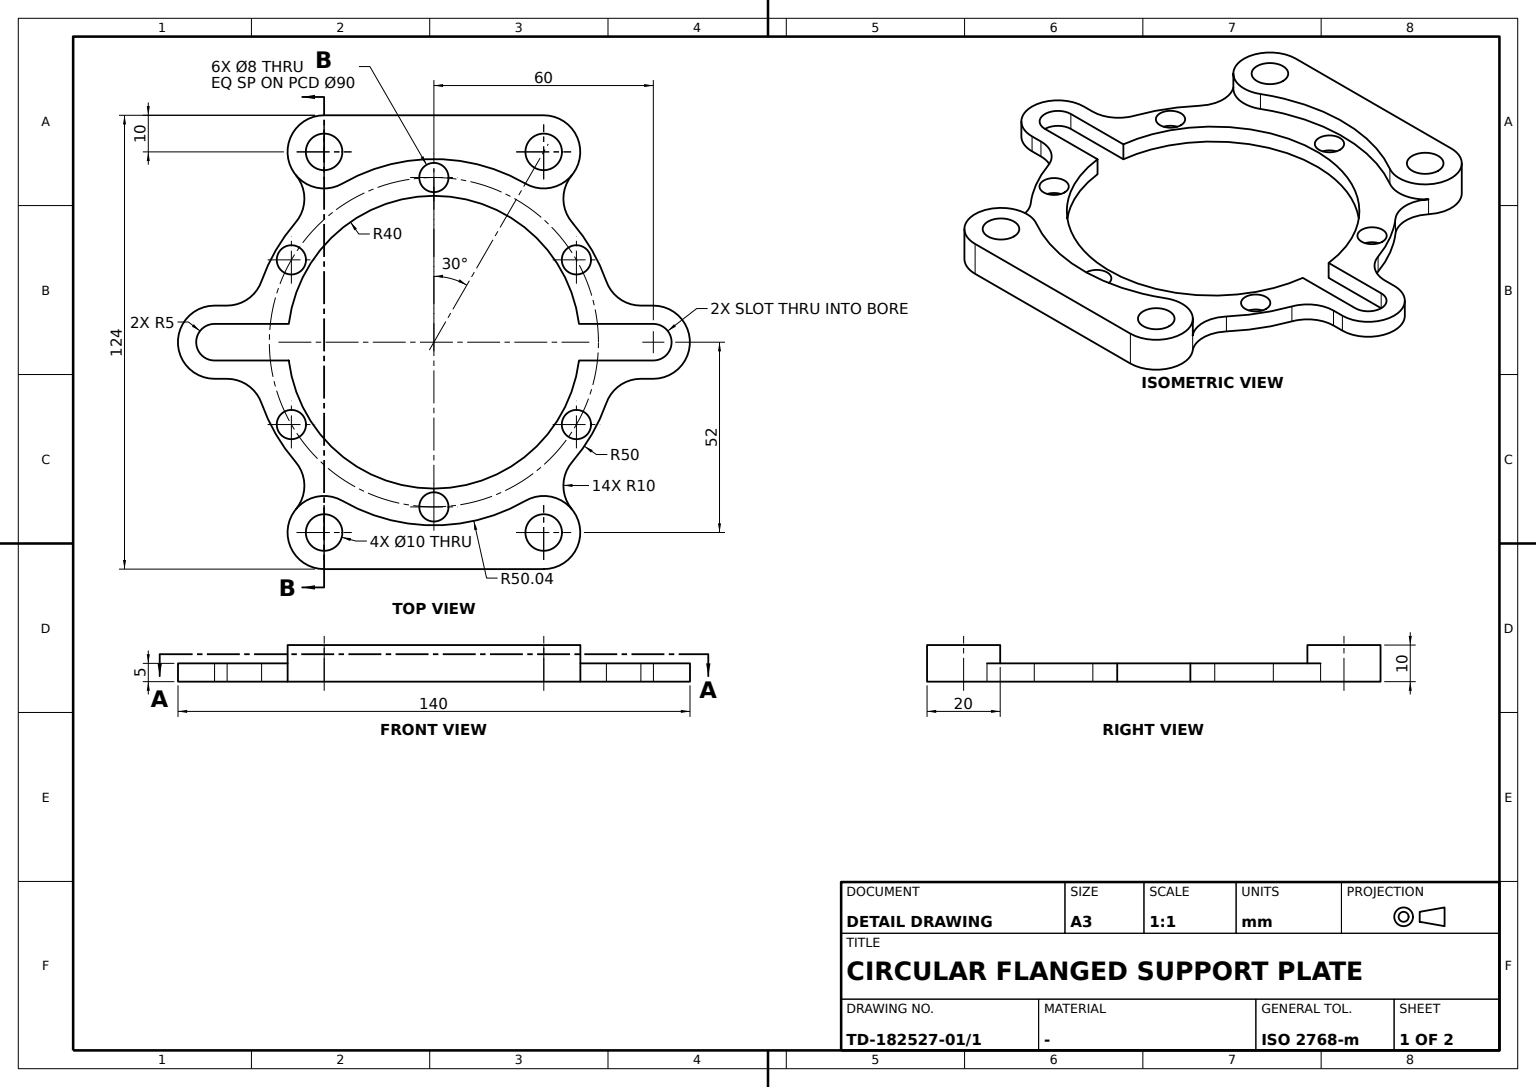
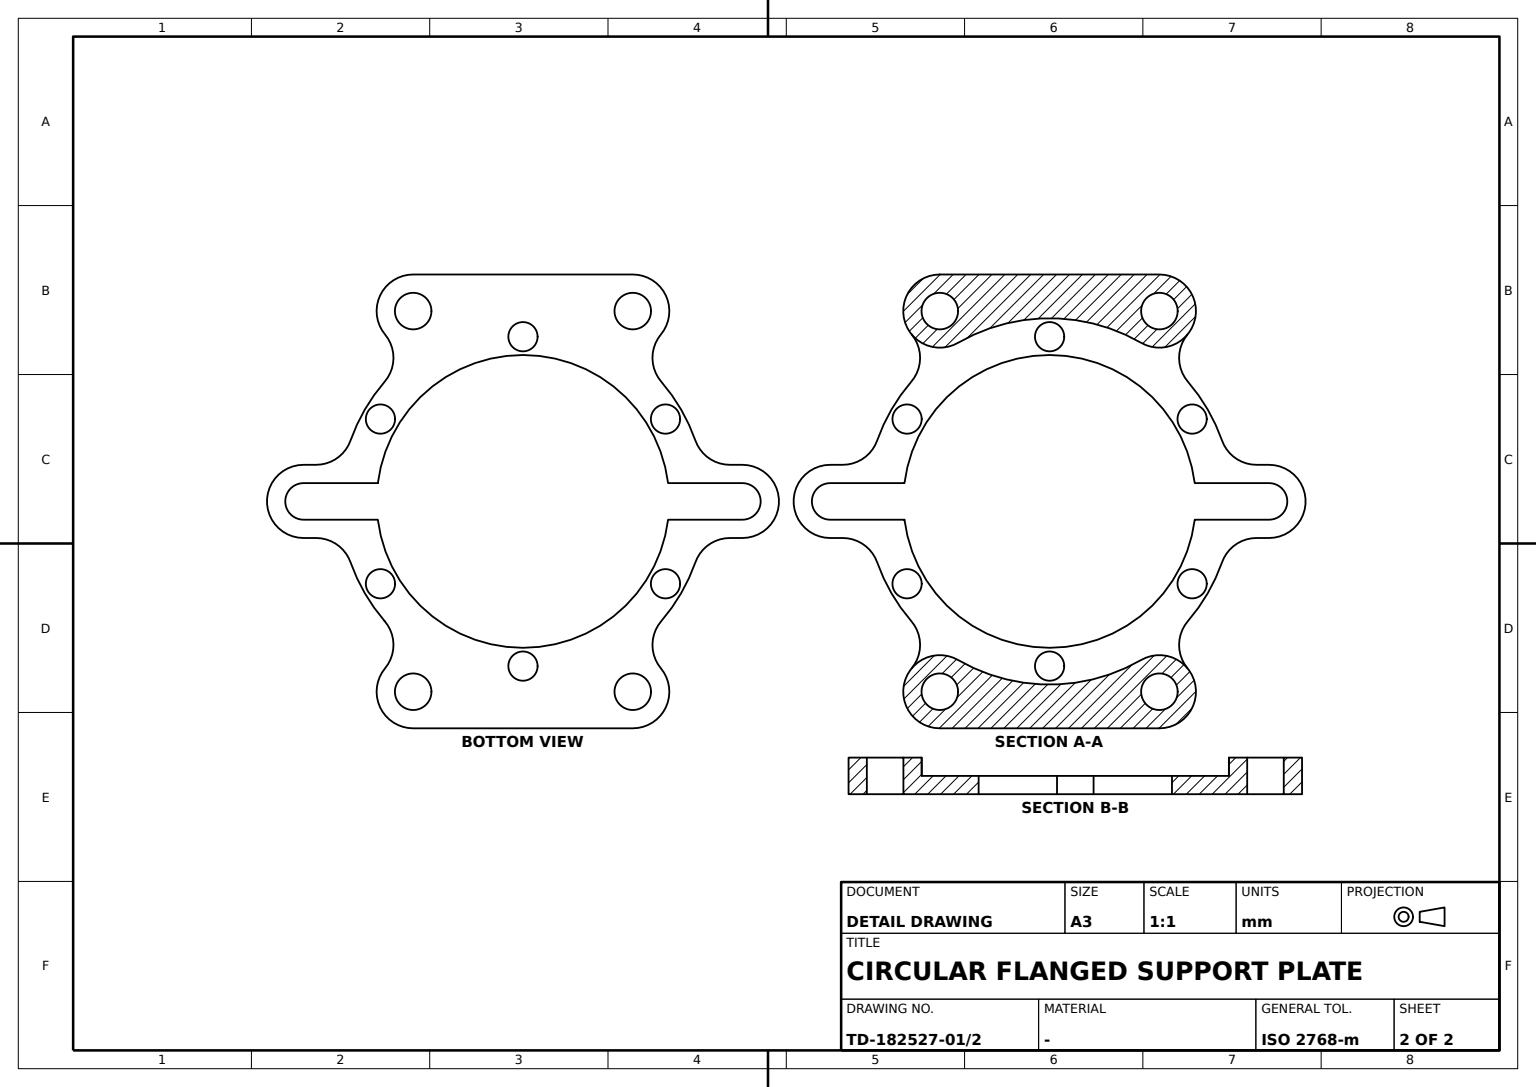
solid
v1 (-25.0222139979,52,5)
e1 v1 v1 CIRCLE(AX(P(-30.0222139979,52,5),D(0,0,1),D(1,0,0)),5)
v2 (-25.0222139979,52,-5)
e2 v2 v2 CIRCLE(AX(P(-30.0222139979,52,-5),D(0,0,1),D(1,0,0)),5)
face CYL(AX(P(-30.0222139979,52,-10),D(0,0,1),D(1,0,0)),5) rev [e1] [-e2]
v3 (-37.8388717769,32.6836317237,0)
v4 (-37.8388717769,32.6836317237,-5)
e3 v3 v4 LINE
v5 (-47.1404520791,16.6666666667,-5)
e4 v4 v5 CIRCLE(AX(P(0,0,-5),D(0,0,1),D(1,0,0)),50)
v6 (-47.1404520791,16.6666666667,0)
e5 v6 v5 LINE
e6 v3 v6 CIRCLE(AX(P(0,0,0),D(0,0,1),D(1,0,0)),50)
face CYL(AX(P(0,0,-2.5),D(0,0,1),D(1,0,0)),50) [e3 e4 -e5 -e6]
v7 (56.5685424949,10,0)
v8 (56.5685424949,10,-5)
e7 v7 v8 LINE
v9 (47.1404520791,16.6666666667,-5)
e8 v9 v8 CIRCLE(AX(P(56.5685424949,20,-5),D(0,0,1),D(1,0,0)),10)
v10 (47.1404520791,16.6666666667,0)
e9 v10 v9 LINE
e10 v10 v7 CIRCLE(AX(P(56.5685424949,20,0),D(0,0,1),D(1,0,0)),10)
face CYL(AX(P(56.5685424949,20,-2.5),D(0,0,1),D(1,0,0)),10) rev [e7 -e8 -e9 e10]
v11 (-39.686269666,-5,0)
v12 (-60,-5,0)
e11 v11 v12 LINE
v13 (-39.686269666,-5,-5)
e12 v11 v13 LINE
v14 (-60,-5,-5)
e13 v13 v14 LINE
e14 v12 v14 LINE
face PLANE(AX(P(60,-5,0),D(0,-1,0),D(-1,0,0))) rev [-e11 e12 e13 -e14]
v15 (37.7144300651,45.6101790342,0)
v16 (37.8388717769,32.6836317237,0)
e15 v15 v16 CIRCLE(AX(P(45.4066461323,39.2203580684,0),D(0,0,1),D(1,0,0)),10)
v17 (37.8388717769,32.6836317237,-5)
e16 v16 v17 LINE
v18 (37.7144300651,45.6101790342,-5)
e17 v18 v17 CIRCLE(AX(P(45.4066461323,39.2203580684,-5),D(0,0,1),D(1,0,0)),10)
e18 v15 v18 LINE
face CYL(AX(P(45.4066461323,39.2203580684,-2.5),D(0,0,1),D(1,0,0)),10) rev [e15 e16 -e17 -e18]
v19 (-60,10,-5)
v20 (-56.5685424949,10,-5)
e19 v19 v20 LINE
v21 (-60,10,0)
e20 v21 v19 LINE
v22 (-56.5685424949,10,0)
e21 v21 v22 LINE
e22 v22 v20 LINE
face PLANE(AX(P(-60,10,0),D(0,1,0),D(1,0,0))) [-e19 -e20 e21 e22]
v23 (37.7144300651,-45.6101790342,0)
v24 (37.7144300651,-45.6101790342,-5)
e23 v23 v24 LINE
v25 (37.8388717769,-32.6836317237,-5)
e24 v25 v24 CIRCLE(AX(P(45.4066461323,-39.2203580684,-5),D(0,0,1),D(1,0,0)),10)
v26 (37.8388717769,-32.6836317237,0)
e25 v26 v25 LINE
e26 v26 v23 CIRCLE(AX(P(45.4066461323,-39.2203580684,0),D(0,0,1),D(1,0,0)),10)
face CYL(AX(P(45.4066461323,-39.2203580684,-2.5),D(0,0,1),D(1,0,0)),10) rev [e23 -e24 -e25 e26]
v27 (60,10,-5)
e27 v8 v27 LINE
v28 (60,10,0)
e28 v7 v28 LINE
e29 v28 v27 LINE
face PLANE(AX(P(-60,10,0),D(0,1,0),D(1,0,0))) [-e27 -e7 e28 e29]
v29 (60,-5,0)
v30 (39.686269666,-5,0)
e30 v29 v30 LINE
v31 (60,-5,-5)
e31 v29 v31 LINE
v32 (39.686269666,-5,-5)
e32 v31 v32 LINE
e33 v30 v32 LINE
face PLANE(AX(P(60,-5,0),D(0,-1,0),D(-1,0,0))) rev [-e30 e31 e32 -e33]
v33 (35.0222139979,52,5)
e34 v33 v33 CIRCLE(AX(P(30.0222139979,52,5),D(0,0,1),D(1,0,0)),5)
v34 (35.0222139979,52,-5)
e35 v34 v34 CIRCLE(AX(P(30.0222139979,52,-5),D(0,0,1),D(1,0,0)),5)
face CYL(AX(P(30.0222139979,52,-10),D(0,0,1),D(1,0,0)),5) rev [e34] [-e35]
v35 (39.686269666,5,-5)
v36 (60,5,-5)
e36 v35 v36 LINE
v37 (60,5,0)
e37 v37 v36 LINE
v38 (39.686269666,5,0)
e38 v38 v37 LINE
e39 v38 v35 LINE
face PLANE(AX(P(39.686269666,5,0),D(0,1,0),D(1,0,0))) rev [e36 -e37 -e38 e39]
v39 (-30.0222139979,-62,5)
v40 (-30.0222139979,-62,-5)
e40 v39 v40 LINE
v41 (30.0222139979,-62,-5)
e41 v40 v41 LINE
v42 (30.0222139979,-62,5)
e42 v42 v41 LINE
e43 v42 v39 LINE
face PLANE(AX(P(-30.0222139979,-62,0),D(0,1,0),D(1,0,0))) rev [e40 e41 -e42 e43]
e44 v41 v24 CIRCLE(AX(P(30.0222139979,-52,-5),D(0,0,1),D(1,0,0)),10)
v43 (25.0222139979,-43.3397459622,0)
e45 v23 v43 CIRCLE(AX(P(30.0222139979,-52,0),D(0,0,1),D(1,0,0)),10)
v44 (25.0222139979,-43.3397459622,5)
e46 v43 v44 LINE
e47 v42 v44 CIRCLE(AX(P(30.0222139979,-52,5),D(0,0,1),D(1,0,0)),10)
face CYL(AX(P(30.0222139979,-52,-2.5),D(0,0,1),D(1,0,0)),10) [e44 -e23 e45 e46 -e47 e42]
v45 (-34.9711431703,22.5,0)
e48 v45 v45 CIRCLE(AX(P(-38.9711431703,22.5,0),D(0,0,1),D(1,0,0)),4)
v46 (42.9711431703,-22.5,0)
e49 v46 v46 CIRCLE(AX(P(38.9711431703,-22.5,0),D(0,0,1),D(1,0,0)),4)
v47 (42.9711431703,22.5,0)
e50 v47 v47 CIRCLE(AX(P(38.9711431703,22.5,0),D(0,0,1),D(1,0,0)),4)
v48 (-34.9711431703,-22.5,0)
e51 v48 v48 CIRCLE(AX(P(-38.9711431703,-22.5,0),D(0,0,1),D(1,0,0)),4)
e52 v10 v16 CIRCLE(AX(P(0,0,0),D(0,0,1),D(1,0,0)),50)
v49 (25.0222139979,43.3397459622,0)
e53 v49 v15 CIRCLE(AX(P(30.0222139979,52,0),D(0,0,1),D(1,0,0)),10)
v50 (-25.0222139979,43.3397459622,0)
e54 v49 v50 CIRCLE(AX(P(0,0,0),D(0,0,1),D(1,0,0)),50.0444279957)
v51 (-37.7144300651,45.6101790342,0)
e55 v51 v50 CIRCLE(AX(P(-30.0222139979,52,0),D(0,0,1),D(1,0,0)),10)
e56 v3 v51 CIRCLE(AX(P(-45.4066461323,39.2203580684,0),D(0,0,1),D(1,0,0)),10)
e57 v22 v6 CIRCLE(AX(P(-56.5685424949,20,0),D(0,0,1),D(1,0,0)),10)
v52 (-60,-10,0)
e58 v21 v52 CIRCLE(AX(P(-60,0,0),D(0,0,1),D(1,0,0)),10)
v53 (-56.5685424949,-10,0)
e59 v53 v52 LINE
v54 (-47.1404520791,-16.6666666667,0)
e60 v54 v53 CIRCLE(AX(P(-56.5685424949,-20,0),D(0,0,1),D(1,0,0)),10)
v55 (-37.8388717769,-32.6836317237,0)
e61 v54 v55 CIRCLE(AX(P(0,0,0),D(0,0,1),D(1,0,0)),50)
v56 (-37.7144300651,-45.6101790342,0)
e62 v56 v55 CIRCLE(AX(P(-45.4066461323,-39.2203580684,0),D(0,0,1),D(1,0,0)),10)
v57 (-25.0222139979,-43.3397459622,0)
e63 v57 v56 CIRCLE(AX(P(-30.0222139979,-52,0),D(0,0,1),D(1,0,0)),10)
e64 v57 v43 CIRCLE(AX(P(0,0,0),D(0,0,1),D(1,0,0)),50.0444279957)
v58 (47.1404520791,-16.6666666667,0)
e65 v26 v58 CIRCLE(AX(P(0,0,0),D(0,0,1),D(1,0,0)),50)
v59 (56.5685424949,-10,0)
e66 v59 v58 CIRCLE(AX(P(56.5685424949,-20,0),D(0,0,1),D(1,0,0)),10)
v60 (60,-10,0)
e67 v60 v59 LINE
e68 v60 v28 CIRCLE(AX(P(60,0,0),D(0,0,1),D(1,0,0)),10)
v61 (-39.686269666,5,0)
e69 v38 v61 CIRCLE(AX(P(0,0,0),D(0,0,1),D(1,0,0)),40)
e70 v29 v37 CIRCLE(AX(P(60,0,0),D(0,0,1),D(1,0,0)),5)
e71 v11 v30 CIRCLE(AX(P(0,0,0),D(0,0,1),D(1,0,0)),40)
v62 (-60,5,0)
e72 v62 v12 CIRCLE(AX(P(-60,0,0),D(0,0,1),D(1,0,0)),5)
e73 v62 v61 LINE
v63 (4,-45,0)
e74 v63 v63 CIRCLE(AX(P(0,-45,0),D(0,0,1),D(1,0,0)),4)
v64 (4,45,0)
e75 v64 v64 CIRCLE(AX(P(0,45,0),D(0,0,1),D(1,0,0)),4)
face PLANE(AX(P(0,0,0),D(0,0,1),D(1,0,0))) [-e48] [-e49] [-e50] [-e51] [-e28 -e10 e52 -e15 -e53 e54 -e55 -e56 e6 -e57 -e21 e58 -e59 -e60 e61 -e62 -e63 e64 -e45 -e26 e65 -e66 -e67 e68] [-e69 e38 -e70 e30 -e71 e11 -e72 e73] [-e74] [-e75]
v65 (-25.0222139979,-52,5)
e76 v65 v65 CIRCLE(AX(P(-30.0222139979,-52,5),D(0,0,1),D(1,0,0)),5)
v66 (-25.0222139979,-52,-5)
e77 v66 v66 CIRCLE(AX(P(-30.0222139979,-52,-5),D(0,0,1),D(1,0,0)),5)
face CYL(AX(P(-30.0222139979,-52,-10),D(0,0,1),D(1,0,0)),5) rev [e76] [-e77]
v67 (25.0222139979,43.3397459622,5)
v68 (30.0222139979,62,5)
e78 v67 v68 CIRCLE(AX(P(30.0222139979,52,5),D(0,0,1),D(1,0,0)),10)
v69 (-30.0222139979,62,5)
e79 v69 v68 LINE
v70 (-25.0222139979,43.3397459622,5)
e80 v69 v70 CIRCLE(AX(P(-30.0222139979,52,5),D(0,0,1),D(1,0,0)),10)
e81 v67 v70 CIRCLE(AX(P(0,0,5),D(0,0,1),D(1,0,0)),50.0444279957)
face PLANE(AX(P(0,0,5),D(0,0,1),D(1,0,0))) [-e1] [e78 -e79 e80 -e81] [-e34]
v71 (42.9711431703,-22.5,-5)
e82 v71 v71 CIRCLE(AX(P(38.9711431703,-22.5,-5),D(0,0,1),D(1,0,0)),4)
face CYL(AX(P(38.9711431703,-22.5,-10),D(0,0,1),D(1,0,0)),4) rev [-e82] [e49]
v72 (-37.8388717769,-32.6836317237,-5)
e83 v55 v72 LINE
v73 (-47.1404520791,-16.6666666667,-5)
e84 v54 v73 LINE
e85 v73 v72 CIRCLE(AX(P(0,0,-5),D(0,0,1),D(1,0,0)),50)
face CYL(AX(P(0,0,-2.5),D(0,0,1),D(1,0,0)),50) [-e83 -e61 e84 e85]
e86 v50 v70 LINE
e87 v49 v67 LINE
face CYL(AX(P(0,0,2.5),D(0,0,1),D(1,0,0)),50.0444279957) rev [e81 -e86 -e54 e87]
v74 (-25.0222139979,-43.3397459622,5)
e88 v57 v74 LINE
e89 v74 v44 CIRCLE(AX(P(0,0,5),D(0,0,1),D(1,0,0)),50.0444279957)
face CYL(AX(P(0,0,2.5),D(0,0,1),D(1,0,0)),50.0444279957) rev [-e64 e88 e89 -e46]
v75 (4,-45,-5)
e90 v75 v75 CIRCLE(AX(P(0,-45,-5),D(0,0,1),D(1,0,0)),4)
face CYL(AX(P(0,-45,-10),D(0,0,1),D(1,0,0)),4) rev [e74] [-e90]
v76 (56.5685424949,-10,-5)
e91 v59 v76 LINE
v77 (60,-10,-5)
e92 v77 v76 LINE
e93 v60 v77 LINE
face PLANE(AX(P(-56.5685424949,-10,0),D(0,-1,0),D(-1,0,0))) [e67 e91 -e92 -e93]
e94 v13 v32 CIRCLE(AX(P(0,0,-5),D(0,0,1),D(1,0,0)),40)
face CYL(AX(P(0,0,-2.5),D(0,0,1),D(1,0,0)),40) rev [e33 -e94 -e12 e71]
v78 (30.0222139979,62,-5)
e95 v68 v78 LINE
v79 (-30.0222139979,62,-5)
e96 v79 v78 LINE
e97 v69 v79 LINE
face PLANE(AX(P(-30.0222139979,62,0),D(0,1,0),D(1,0,0))) [e95 -e96 -e97 e79]
e98 v77 v27 CIRCLE(AX(P(60,0,-5),D(0,0,1),D(1,0,0)),10)
face CYL(AX(P(60,0,-2.5),D(0,0,1),D(1,0,0)),10) [e98 -e29 -e68 e93]
v80 (4,45,-5)
e99 v80 v80 CIRCLE(AX(P(0,45,-5),D(0,0,1),D(1,0,0)),4)
face CYL(AX(P(0,45,-10),D(0,0,1),D(1,0,0)),4) rev [e75] [-e99]
v81 (-60,-10,-5)
e100 v19 v81 CIRCLE(AX(P(-60,0,-5),D(0,0,1),D(1,0,0)),10)
e101 v52 v81 LINE
face CYL(AX(P(-60,0,-2.5),D(0,0,1),D(1,0,0)),10) [e20 e100 -e101 -e58]
e102 v31 v36 CIRCLE(AX(P(60,0,-5),D(0,0,1),D(1,0,0)),5)
face CYL(AX(P(60,0,-2.5),D(0,0,1),D(1,0,0)),5) rev [-e31 e70 e37 -e102]
v82 (47.1404520791,-16.6666666667,-5)
e103 v25 v82 CIRCLE(AX(P(0,0,-5),D(0,0,1),D(1,0,0)),50)
e104 v58 v82 LINE
face CYL(AX(P(0,0,-2.5),D(0,0,1),D(1,0,0)),50) [-e65 e25 e103 -e104]
e105 v9 v17 CIRCLE(AX(P(0,0,-5),D(0,0,1),D(1,0,0)),50)
face CYL(AX(P(0,0,-2.5),D(0,0,1),D(1,0,0)),50) [e9 e105 -e16 -e52]
v83 (35.0222139979,-52,-5)
e106 v83 v83 CIRCLE(AX(P(30.0222139979,-52,-5),D(0,0,1),D(1,0,0)),5)
v84 (35.0222139979,-52,5)
e107 v84 v84 CIRCLE(AX(P(30.0222139979,-52,5),D(0,0,1),D(1,0,0)),5)
face CYL(AX(P(30.0222139979,-52,-10),D(0,0,1),D(1,0,0)),5) rev [-e106] [e107]
v85 (42.9711431703,22.5,-5)
e108 v85 v85 CIRCLE(AX(P(38.9711431703,22.5,-5),D(0,0,1),D(1,0,0)),4)
face CYL(AX(P(38.9711431703,22.5,-10),D(0,0,1),D(1,0,0)),4) rev [e50] [-e108]
v86 (-60,5,-5)
v87 (-39.686269666,5,-5)
e109 v86 v87 LINE
e110 v61 v87 LINE
e111 v62 v86 LINE
face PLANE(AX(P(39.686269666,5,0),D(0,1,0),D(1,0,0))) rev [e109 -e110 -e73 e111]
e112 v76 v82 CIRCLE(AX(P(56.5685424949,-20,-5),D(0,0,1),D(1,0,0)),10)
face CYL(AX(P(56.5685424949,-20,-2.5),D(0,0,1),D(1,0,0)),10) rev [e104 -e112 -e91 e66]
e113 v35 v87 CIRCLE(AX(P(0,0,-5),D(0,0,1),D(1,0,0)),40)
face CYL(AX(P(0,0,-2.5),D(0,0,1),D(1,0,0)),40) rev [e69 e110 -e113 -e39]
v88 (-37.7144300651,-45.6101790342,-5)
e114 v88 v72 CIRCLE(AX(P(-45.4066461323,-39.2203580684,-5),D(0,0,1),D(1,0,0)),10)
e115 v56 v88 LINE
face CYL(AX(P(-45.4066461323,-39.2203580684,-2.5),D(0,0,1),D(1,0,0)),10) rev [-e114 -e115 e62 e83]
e116 v86 v14 CIRCLE(AX(P(-60,0,-5),D(0,0,1),D(1,0,0)),5)
face CYL(AX(P(-60,0,-2.5),D(0,0,1),D(1,0,0)),5) rev [-e116 -e111 e72 e14]
v89 (-34.9711431703,22.5,-5)
e117 v89 v89 CIRCLE(AX(P(-38.9711431703,22.5,-5),D(0,0,1),D(1,0,0)),4)
face CYL(AX(P(-38.9711431703,22.5,-10),D(0,0,1),D(1,0,0)),4) rev [e48] [-e117]
e118 v88 v40 CIRCLE(AX(P(-30.0222139979,-52,-5),D(0,0,1),D(1,0,0)),10)
v90 (-56.5685424949,-10,-5)
e119 v73 v90 CIRCLE(AX(P(-56.5685424949,-20,-5),D(0,0,1),D(1,0,0)),10)
e120 v90 v81 LINE
e121 v20 v5 CIRCLE(AX(P(-56.5685424949,20,-5),D(0,0,1),D(1,0,0)),10)
v91 (-37.7144300651,45.6101790342,-5)
e122 v4 v91 CIRCLE(AX(P(-45.4066461323,39.2203580684,-5),D(0,0,1),D(1,0,0)),10)
e123 v79 v91 CIRCLE(AX(P(-30.0222139979,52,-5),D(0,0,1),D(1,0,0)),10)
e124 v18 v78 CIRCLE(AX(P(30.0222139979,52,-5),D(0,0,1),D(1,0,0)),10)
v92 (-34.9711431703,-22.5,-5)
e125 v92 v92 CIRCLE(AX(P(-38.9711431703,-22.5,-5),D(0,0,1),D(1,0,0)),4)
face PLANE(AX(P(0,0,-5),D(0,0,1),D(1,0,0))) rev [-e32 e102 -e36 e113 -e109 e116 -e13 e94] [e35] [e92 e112 -e103 e24 -e44 -e41 -e118 e114 -e85 e119 e120 -e100 e19 e121 -e4 e122 -e123 e96 -e124 e17 -e105 e8 e27 -e98] [e106] [e90] [e125] [e99] [e82] [e117] [e108] [e2] [e77]
e126 v51 v91 LINE
face CYL(AX(P(-45.4066461323,39.2203580684,-2.5),D(0,0,1),D(1,0,0)),10) rev [e126 -e122 -e3 e56]
e127 v74 v39 CIRCLE(AX(P(-30.0222139979,-52,5),D(0,0,1),D(1,0,0)),10)
face CYL(AX(P(-30.0222139979,-52,-2.5),D(0,0,1),D(1,0,0)),10) [-e88 e63 e115 e118 -e40 -e127]
e128 v53 v90 LINE
face CYL(AX(P(-56.5685424949,-20,-2.5),D(0,0,1),D(1,0,0)),10) rev [-e119 -e84 e60 e128]
face CYL(AX(P(-30.0222139979,52,-2.5),D(0,0,1),D(1,0,0)),10) [e55 e86 -e80 e97 e123 -e126]
face CYL(AX(P(30.0222139979,52,-2.5),D(0,0,1),D(1,0,0)),10) [-e78 -e87 e53 e18 e124 -e95]
face PLANE(AX(P(0,0,5),D(0,0,1),D(1,0,0))) [-e76] [e47 -e89 e127 -e43] [-e107]
face CYL(AX(P(-38.9711431703,-22.5,-10),D(0,0,1),D(1,0,0)),4) rev [e51] [-e125]
face PLANE(AX(P(-56.5685424949,-10,0),D(0,-1,0),D(-1,0,0))) [-e128 e59 e101 -e120]
face CYL(AX(P(-56.5685424949,20,-2.5),D(0,0,1),D(1,0,0)),10) rev [e57 e5 -e121 -e22]
